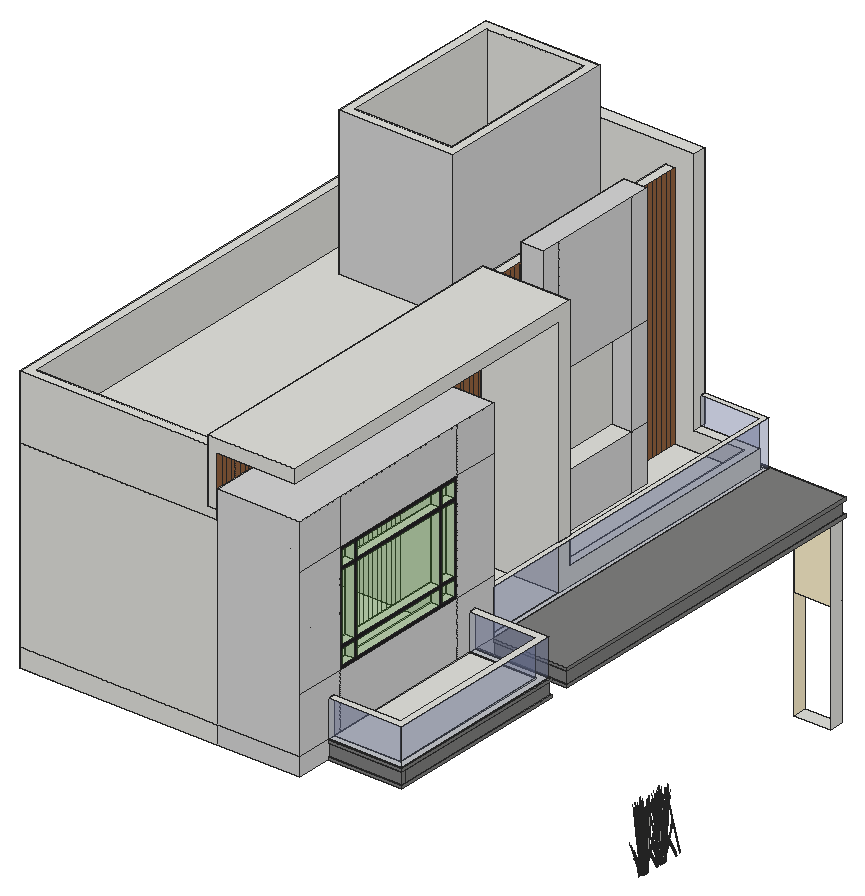
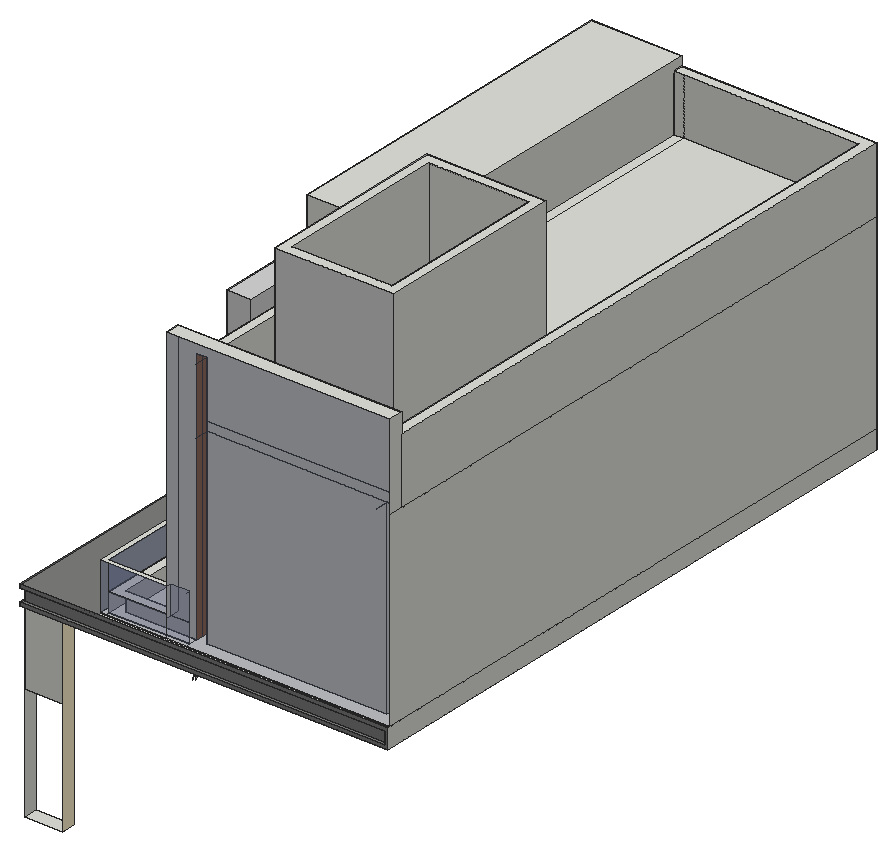
# SketchUp Ruby script. Lengths in inches.
U = 1.inch
M = Sketchup.active_model
def pt(a) = Geom::Point3d.new(a.map { |v| v * U })
def face(e, loops, mat)
  f = e.add_face(loops[0].map { |a| pt(a) })
  loops[1..].each { |l| e.add_face(l.map { |a| pt(a) }).erase! }
  f.material = f.back_material = mat if mat
  f
end
# faces: each face lists its corners as indices into pts; further lists are holes
def faces(e, pts, list, mat = nil) = list.each { |f| face(e, (f[0].is_a?(Array) ? f : [f]).map { |l| l.map { |i| pts[i] } }, mat) }
# xy, xz, yz: faces in a plane at the given z, y or x. An outline is a flat list of corners, or four numbers for a rectangle; further outlines are holes
def ring(l) = l.size == 4 ? [[l[0], l[1]], [l[2], l[1]], [l[2], l[3]], [l[0], l[3]]] : l.each_slice(2).to_a
def flat(e, list, mat, &to3) = list.each { |f| face(e, (f[0].is_a?(Array) ? f : [f]).map { |l| ring(l).map { |u, v| to3.(u, v) } }, mat) }
def xy(e, z, list, mat = nil) = flat(e, list, mat) { |x, y| [x, y, z] }
def xz(e, y, list, mat = nil) = flat(e, list, mat) { |x, z| [x, y, z] }
def yz(e, x, list, mat = nil) = flat(e, list, mat) { |y, z| [x, y, z] }
def lines(e, pts, list) = list.each { |a, b| e.add_line(pt(pts[a]), pt(pts[b])) }
# prism: a flat outline (further loops are holes) pulled along v
def prism(e, loops, v, mat = nil)
  f = face(e, loops, mat); d = Geom::Vector3d.new(v.map { |x| x * U })
  f.pushpull(f.normal.samedirection?(d) ? d.length : -d.length)
end
def box(e, o, s, mat = nil) = prism(e, [[o, [o[0] + s[0], o[1], o[2]], [o[0] + s[0], o[1] + s[1], o[2]], [o[0], o[1] + s[1], o[2]]]], [0, 0, s[2]], mat)
def at(x, y, z, deg = 0) = Geom::Transformation.translation(pt([x, y, z])) * Geom::Transformation.rotation(ORIGIN, Z_AXIS, deg.degrees)
def axes(o, x, y, z) = Geom::Transformation.new([*x, 0, *y, 0, *z, 0, *pt(o).to_a, 1])
def part(name) = M.definitions.add(name)
# library, detail: a bought-in or finely detailed component or shape, given as its bounding box
def library(name, o, s) = part(name).tap { |d| box(d.entities, o, s) }
def detail(e, o, s) = box(e.add_group.entities, o, s)
def put(e, d, t, mat = nil) = e.add_instance(d, t).tap { |i| i.material = mat if mat }
def group(e, t, mat = nil) = e.add_group.tap { |g| g.transformation = t; g.material = mat if mat }.entities
root = M.entities
M.materials.add("D01_Frost_White").color = [255, 242, 206]
M.materials.add("Glass_Basic_01").color = [81, 188, 38]
M.materials["Glass_Basic_01"].alpha = 0.25
M.materials.add("Glass_Sky Reflection_01").color = [126, 138, 183]
M.materials["Glass_Sky Reflection_01"].alpha = 0.25
M.materials.add("LightPink_Translucent").color = [144, 107, 117]
M.materials["LightPink_Translucent"].alpha = 0.75
M.materials.add("Marble_07_1K").color = [36, 34, 36]
M.materials.add("ThomThom - Waistcoat1").color = [214, 214, 214]
M.materials.add("ThomThom - Waistcoat2").color = [127, 127, 126]
M.materials.add("Wood_Veneer_15_1K").color = [150, 100, 65]
M.materials.add("wheel_emblem1").color = [204, 204, 204]
c1 = part("blade")
p = [[2.15,0.21,22],[0,0.17,0],[0.09,0.45,0],[2.18,0.31,22],[2.29,0.31,22],[0.38,0.45,0],
  [2.48,0.24,33],[2.49,0.24,33],[2.48,0.22,33]]
faces(c1.entities,p,[[0,1,2,3],[4,5,2,3],[6,3,4,7],[8,0,3,6]])
c2 = part("seeds")
p = [[0.3,-0.1,1.38],[-0.01,-0.03,1.59],[-0.01,-0.03,0.03],[0.14,-0.07,-0.07],[0.29,-0.03,3],[0.15,0.01,3.11]]
faces(c2.entities,p,[[0,1,2,3],[1,0,4,5]],"LightPink_Translucent")
c3 = part("blade with seeds")
put(c3.entities,c1,at(0,0,0))
put(c3.entities,c2,axes([2.4,0.25,30.99],[1.5799,-0.05474,1.17369],[-0.12525,1.92788,0.29478],[-0.07173,-0.02425,1.56792]))
g1 = group(root,at(0,1.43,120))
xy(g1,-120,[[207,375,231,384]])
xy(g1,0,[[207,375,231,384],[231,375,232,386],[207,384,231,386]])
xy(g1,0,[[0,0,183,24],[183,23,183,24,0,24,0,146.4,183,146.4,183,145,232,145,232,23],[0,146.4,183,150],[0,150,183,153.6],[0,153.6,183,157.2],
  [0,157.2,0,376.8,207,376.8,207,375,232,375,232,158,183,158,183,157.2],[0,376.8,207,380.4],[0,380.4,207,386]],"Wood_Veneer_15_1K")
xy(g1,2,[[183,23,231,24],[231,23,232,26],[231,26,232,145],[183,144,231,145],[231,158,232,158,232,386,2,386,2,384,231,384],
  [183,158,231,159]],"ThomThom - Waistcoat2")
xy(g1,6,[[183,28.5,226.5,139.5]])
xy(g1,10,[[183,23,231,24],[231,23,232,26]])
xy(g1,10,[[231,26,232,145],[183,144,231,145],[183,158,231,159],[231,158,232,386],[2,384,231,386]],"ThomThom - Waistcoat2")
xy(g1,12,[[[0,0,183,0,183,159,129,159,129,225,174,225,174,375,129,375,129,384,0,384],[129,249,144,333]],[183,24,231,24,231,144,183,144,183,139.5,226.5,139.5,226.5,28.5,183,28.5],[183,28.5,226.5,139.5],[129,159,180,216],[180,159,183,384],
  [129,216,180,216,180,249,174,249,174,225,129,225],[129,249,144,333],[174,249,180,333],[174,333,180,333,180,381,129,381,129,375,174,375],[129,381,180,384],
  [0,384,129,386],[129,384,141,386],[141,384,180,386],[180,384,183,386]])
xy(g1,12,[[183,23,231,24],[231,23,232,145],[183,144,231,145],[183,158,232,386]],"ThomThom - Waistcoat2")
xy(g1,24,[[174,225,180,225,180,381,141,381,141,375,174,375]])
xy(g1,36,[[183,24,231,24,231,144,183,144,183,139.5,226.5,139.5,226.5,28.5,183,28.5]])
xy(g1,42,[[180,159,183,159,183,384,141,384,141,381,180,381]])
xy(g1,48,[[129,261,130.78,321],[130.78,261,144,321]])
xy(g1,50,[[177,35,183,45],[177,47,183,115],[177,117,183,127]])
xy(g1,60,[[177,35,183,45],[177,47,183,115],[177,117,183,127]])
xy(g1,62,[[177,35,183,45],[177,47,183,115],[177,117,183,127]])
xy(g1,106,[[177,35,183,45],[177,47,183,115],[177,117,183,127]])
xy(g1,108,[[177,35,183,45],[177,47,183,115],[177,117,183,127],[129,261,130.78,321],[130.78,261,144,321]])
xy(g1,118,[[177,35,183,45],[177,47,183,115],[177,117,183,127]])
xy(g1,132,[[0,0,0,159,129,159,129,153,9,153,9,9,129,9,129,0],[9,9,129,153],[129,9,177,153],[0,159,9,375],[9,159,123,375]])
xy(g1,138,[[123,0,129,159],[117,6,123,6,123,375,6,375,6,369,117,369],[[6,6,117,369],[24,231,99,351]],[30,237,93,345]])
xy(g1,150,[[129,0,183,159]],"ThomThom - Waistcoat1")
xy(g1,171,[[129,0,180,216]],"Wood_Veneer_15_1K")
xy(g1,174,[[0,0,123,0,123,6,6,6,6,375,0,375],[123,225,129,375]])
xy(g1,180,[[123,0,180,225]])
xy(g1,186,[[0,375,141,384]])
xy(g1,186,[[129,249,144,333]],"ThomThom - Waistcoat1")
xy(g1,234,[[[24,231,99,351],[30,237,93,345]]])
xz(g1,0,[[0,0,129,12],[0,12,129,132],[0,132,129,132,129,138,123,138,123,174,0,174],[123,138,129,138,129,171,180,171,180,180,123,180]])
xz(g1,0,[[129,0,183,12],[129,12,183,150]],"ThomThom - Waistcoat1")
xz(g1,6,[[6,138,117,174],[117,138,123,174]])
xz(g1,9,[[9,12,177,132]])
xz(g1,23,[[183,0,232,2],[183,10,232,12]],"ThomThom - Waistcoat2")
xz(g1,24,[[183,12,231,36]],"Glass_Sky Reflection_01")
xz(g1,24,[[183,2,231,10]],"ThomThom - Waistcoat2")
xz(g1,28.5,[[183,6,226.5,12]])
xz(g1,28.5,[[183,12,226.5,36]],"Glass_Sky Reflection_01")
xz(g1,35,[[177,50,183,60],[177,62,183,106],[177,108,183,118]])
xz(g1,45,[[177,50,183,60],[177,62,183,106],[177,108,183,118]])
xz(g1,47,[[177,50,183,60],[177,62,183,106],[177,108,183,118]])
xz(g1,115,[[177,50,183,60],[177,62,183,106],[177,108,183,118]])
xz(g1,117,[[177,50,183,60],[177,62,183,106],[177,108,183,118]])
xz(g1,127,[[177,50,183,60],[177,62,183,106],[177,108,183,118]])
xz(g1,139.5,[[183,6,226.5,12]])
xz(g1,139.5,[[183,12,226.5,36]],"Glass_Sky Reflection_01")
xz(g1,144,[[183,12,231,36]],"Glass_Sky Reflection_01")
xz(g1,144,[[183,2,231,10]],"ThomThom - Waistcoat2")
xz(g1,145,[[183,0,232,2],[183,10,232,12]],"ThomThom - Waistcoat2")
xz(g1,153,[[9,12,177,132]])
xz(g1,158,[[183,0,232,2],[183,10,232,12]],"ThomThom - Waistcoat2")
xz(g1,159,[[9,12,123,132],[180,12,183,42],[123,132,129,138]])
xz(g1,159,[[129,12,129,150,183,150,183,42,180,42,180,12]],"ThomThom - Waistcoat1")
xz(g1,159,[[183,2,231,10]],"ThomThom - Waistcoat2")
xz(g1,216,[[129,12,180,171]])
xz(g1,225,[[129,12,129,174,123,174,123,180,180,180,180,24,174,24,174,12]])
xz(g1,231,[[24,138,99,234]],"ThomThom - Waistcoat1")
xz(g1,237,[[30,138,93,234]])
xz(g1,249,[[129,12,144,186]],"ThomThom - Waistcoat1")
xz(g1,261,[[129,48,130.78,108]])
xz(g1,261,[[130.78,48,144,108]],"ThomThom - Waistcoat1")
xz(g1,321,[[129,48,130.78,108]])
xz(g1,321,[[130.78,48,144,108]],"ThomThom - Waistcoat1")
xz(g1,333,[[129,12,144,186]],"ThomThom - Waistcoat1")
xz(g1,345,[[30,138,93,234]])
xz(g1,351,[[24,138,99,234]],"ThomThom - Waistcoat1")
xz(g1,375,[[129,12,174,12,174,24,141,24,141,186,0,186,0,174,6,174,6,138,123,138,123,174,129,174],[9,12,123,132],[0,132,123,132,123,138,6,138,6,174,0,174]])
xz(g1,375,[[207,-47.78,231,0]],"D01_Frost_White")
xz(g1,381,[[129,12,180,24],[129,24,141,42],[141,24,180,42]],"Glass_Sky Reflection_01")
xz(g1,384,[[207,-48,231,0]])
xz(g1,384,[[0,12,141,186],[141,12,183,42]],"Glass_Sky Reflection_01")
xz(g1,384,[[2,2,231,10]],"ThomThom - Waistcoat2")
xz(g1,386,[[0,0,0,12,232,12,232,10,2,10,2,2,232,2,232,0]],"ThomThom - Waistcoat2")
yz(g1,0,[[0,0,386,12],[0,12,384,132],[0,132,375,174],[375,132,384,186]])
yz(g1,2,[[384,2,386,10]],"ThomThom - Waistcoat2")
yz(g1,6,[[6,138,369,174],[369,138,375,174]])
yz(g1,9,[[9,12,153,132],[159,12,375,132]])
yz(g1,24,[[231,138,351,234]])
yz(g1,30,[[237,138,345,234]])
yz(g1,93,[[237,138,345,234]])
yz(g1,99,[[231,138,351,234]],"ThomThom - Waistcoat1")
yz(g1,123,[[159,12,375,132],[159,132,375,138],[0,138,6,174],[6,138,6,174,0,174,0,180,225,180,225,174,375,174,375,138]])
yz(g1,129,[[216,12,225,174],[249,12,262.5,12,262.5,48,261,48,261,108,321,108,321,48,318.75,48,318.75,12,333,12,333,174,249,174],[262.5,12,266.25,48],[266.25,12,270,48],[270,12,273.75,48],
  [273.75,12,277.5,48],[277.5,12,281.25,48],[281.25,12,285,48],[285,12,288.75,48],[288.75,12,292.5,48],
  [292.5,12,296.25,48],[296.25,12,300,48],[300,12,303.75,48],[303.75,12,307.5,48],[307.5,12,311.25,48],
  [311.25,12,315,48],[315,12,318.75,48],[0,132,3.75,138],[3.75,132,7.5,138],[7.5,132,11.25,138],
  [11.25,132,15,138],[15,132,18.75,138],[18.75,132,22.5,138],[22.5,132,26.25,138],[26.25,132,30,138],
  [30,132,33.75,138],[33.75,132,37.5,138],[37.5,132,41.25,138],[41.25,132,45,138],[45,132,48.75,138],
  [48.75,132,52.5,138],[52.5,132,56.25,138],[56.25,132,60,138],[60,132,63.75,138],[63.75,132,67.5,138],
  [67.5,132,71.25,138],[71.25,132,75,138],[75,132,78.75,138],[78.75,132,82.5,138],[82.5,132,86.25,138],
  [86.25,132,90,138],[90,132,93.75,138],[93.75,132,97.5,138],[97.5,132,101.25,138],[101.25,132,105,138],
  [105,132,108.75,138],[108.75,132,112.5,138],[112.5,132,116.25,138],[116.25,132,120,138],[120,132,123.75,138],
  [123.75,132,127.5,138],[127.5,132,131.25,138],[131.25,132,135,138],[135,132,138.75,138],[138.75,132,142.5,138],
  [142.5,132,146.25,138],[146.25,132,150,138],[150,132,153.75,138],[153.75,132,157.5,138],[157.5,132,159,138],
  [0,138,3.75,150],[3.75,138,7.5,150],[7.5,138,11.25,150],[11.25,138,15,150],[15,138,18.75,150],
  [18.75,138,22.5,150],[22.5,138,26.25,150],[26.25,138,30,150],[30,138,33.75,150],[33.75,138,37.5,150],
  [37.5,138,41.25,150],[41.25,138,45,150],[45,138,48.75,150],[48.75,138,52.5,150],[52.5,138,56.25,150],
  [56.25,138,60,150],[60,138,63.75,150],[63.75,138,67.5,150],[67.5,138,71.25,150],[71.25,138,75,150],
  [75,138,78.75,150],[78.75,138,82.5,150],[82.5,138,86.25,150],[86.25,138,90,150],[90,138,93.75,150],
  [93.75,138,97.5,150],[97.5,138,101.25,150],[101.25,138,105,150],[105,138,108.75,150],[108.75,138,112.5,150],
  [112.5,138,116.25,150],[116.25,138,120,150],[120,138,123.75,150],[123.75,138,127.5,150],[127.5,138,131.25,150],
  [131.25,138,135,150],[135,138,138.75,150],[138.75,138,142.5,150],[142.5,138,146.25,150],[146.25,138,150,150],
  [150,138,153.75,150],[153.75,138,157.5,150],[157.5,138,159,150]])
yz(g1,129,[[249,174,333,186]],"ThomThom - Waistcoat1")
yz(g1,129,[[159,12,161.25,12,161.25,171,157.5,171,157.5,150,159,150],[161.25,12,165,171],[165,12,168.75,171],[168.75,12,172.5,171],[172.5,12,176.25,171],
  [176.25,12,180,171],[180,12,183.75,171],[183.75,12,187.5,171],[187.5,12,191.25,171],[191.25,12,195,171],
  [195,12,198.75,171],[198.75,12,202.5,171],[202.5,12,206.25,171],[206.25,12,210,171],[210,12,213.75,171],
  [213.75,12,216,171],[225,12,249,174],[333,12,375,174],[0,150,3.75,171],[3.75,150,7.5,171],
  [7.5,150,11.25,171],[11.25,150,15,171],[15,150,18.75,171],[18.75,150,22.5,171],[22.5,150,26.25,171],
  [26.25,150,30,171],[30,150,33.75,171],[33.75,150,37.5,171],[37.5,150,41.25,171],[41.25,150,45,171],
  [45,150,48.75,171],[48.75,150,52.5,171],[52.5,150,56.25,171],[56.25,150,60,171],[60,150,63.75,171],
  [63.75,150,67.5,171],[67.5,150,71.25,171],[71.25,150,75,171],[75,150,78.75,171],[78.75,150,82.5,171],
  [82.5,150,86.25,171],[86.25,150,90,171],[90,150,93.75,171],[93.75,150,97.5,171],[97.5,150,101.25,171],
  [101.25,150,105,171],[105,150,108.75,171],[108.75,150,112.5,171],[112.5,150,116.25,171],[116.25,150,120,171],
  [120,150,123.75,171],[123.75,150,127.5,171],[127.5,150,131.25,171],[131.25,150,135,171],[135,150,138.75,171],
  [138.75,150,142.5,171],[142.5,150,146.25,171],[146.25,150,150,171],[150,150,153.75,171],[153.75,150,157.5,171]],"Wood_Veneer_15_1K")
yz(g1,130.78,[[261,48,321,108]])
yz(g1,141,[[375,24,381,24,381,42,384,42,384,186,375,186],[381,24,384,42]])
yz(g1,144,[[249,12,261,48],[261,12,321,48],[321,12,333,48],[249,48,261,108],[321,48,333,108],
  [249,108,261,186],[261,108,321,186],[321,108,333,186]],"ThomThom - Waistcoat1")
yz(g1,174,[[225,12,375,24]])
yz(g1,177,[[[9,12,153,132],[47,62,115,62,115,106,47,106,47,108,115,108,115,118,47,118],[47,50,115,60],[35,62,45,106],[117,62,127,106],[35,108,45,118],[117,108,127,118],[117,50,127,60],[35,50,45,60]]])
yz(g1,180,[[216,12,381,12,381,24,225,24,225,42,216,42],[216,42,225,42,225,180,0,180,0,171,216,171]])
yz(g1,180,[[159,12,216,42],[225,24,381,42]],"Glass_Sky Reflection_01")
yz(g1,183,[[28.5,6,139.5,12],[24,12,28.5,36],[139.5,12,144,36]])
yz(g1,183,[[35,50,45,60],[47,50,115,60],[117,50,127,60],[35,62,45,106],[47,62,115,106],
  [117,62,127,106],[35,108,45,118],[47,108,115,118],[117,108,127,118]],"Glass_Basic_01")
yz(g1,183,[[159,12,384,42]],"Glass_Sky Reflection_01")
yz(g1,183,[[[33,48,129,120],[47,62,115,106],[35,50,35,118,127,118,127,50,47,50,47,60,115,60,115,50,117,50,117,60,127,60,127,62,117,62,117,106,127,106,127,108,117,108,117,118,115,118,115,108,47,108,47,118,45,118,45,108,35,108,35,106,45,106,45,62,35,62,35,60,45,60,45,50]]],"Marble_07_1K")
yz(g1,183,[[0,0,23,0,23,2,24,2,24,10,23,10,23,12,0,12],[0,12,24,12,24,36,28.5,36,28.5,12,33,12,33,48,0,48],[33,12,129,48],[129,12,139.5,12,139.5,36,144,36,144,12,159,12,159,48,129,48],[0,48,33,120],
  [129,48,159,120],[0,120,33,150],[33,120,129,150],[129,120,159,150]],"ThomThom - Waistcoat1")
yz(g1,183,[[145,0,158,0,158,2,159,2,159,10,158,10,158,12,145,12,145,10,144,10,144,2,145,2]],"wheel_emblem1")
yz(g1,207,[[375,-120,384,0]],"D01_Frost_White")
yz(g1,226.5,[[28.5,6,139.5,12]])
yz(g1,226.5,[[28.5,12,139.5,36]],"Glass_Sky Reflection_01")
yz(g1,231,[[375,-120,384,0]])
yz(g1,231,[[24,12,144,36]],"Glass_Sky Reflection_01")
yz(g1,231,[[24,2,26,10],[26,2,144,10],[159,2,384,10]],"ThomThom - Waistcoat2")
yz(g1,232,[[23,0,145,2],[158,0,386,2],[23,10,145,12],[158,10,386,12]],"ThomThom - Waistcoat2")
p = [[177,9,12],[183,9,12],[129,159,138],[129.2,159,138],[129,381,42],[129,384,42],
  [122.18,159,138],[123,159,138],[123,375,174],[123,384,174],[123,375,132],[123,384,132],
  [9,384,132],[9,375,132],[177,9,84],[183,9,84],[180,219,12],[180.01,219,12],
  [177,9,132],[177,0,132],[177,47,108],[177,45,108],[177,47,106],[177,45,106],
  [231,384,-48],[207,375,-47.78],[129,371.25,11.97],[129,371.25,12],[129,371.25,173.97],[129,367.5,11.94],
  [129,367.5,12],[129,367.5,173.94],[129,363.75,11.91],[129,363.75,12],[129,363.75,173.91],[129,360,11.88],
  [129,360,12],[129,360,173.88],[129,356.25,11.85],[129,356.25,12],[129,356.25,173.85],[129,352.5,11.82],
  [129,352.5,12],[129,352.5,173.82],[129,348.75,11.79],[129,348.75,12],[129,348.75,173.79],[129,345,11.76],
  [129,345,12],[129,345,173.76],[129,341.25,11.73],[129,341.25,12],[129,341.25,173.73],[129,337.5,11.7],
  [129,337.5,12],[129,337.5,173.7],[129,333.75,11.67],[129,333.75,12],[129,333.75,173.67],[129,330,11.64],
  [129,330,12],[129,330,173.64],[129,326.25,11.61],[129,326.25,12],[129,326.25,173.61],[129,322.5,11.58],
  [129,322.5,12],[129,322.5,173.58],[129,318.75,11.55],[129,318.75,12],[129,318.75,48],[129,318.75,108],
  [129,318.75,173.55],[129,315,11.52],[129,315,12],[129,315,48],[129,315,108],[129,315,173.52],
  [129,311.25,11.49],[129,311.25,12],[129,311.25,108],[129,311.25,173.49],[129,311.25,48],[129,307.5,11.46],
  [129,307.5,12],[129,307.5,108],[129,307.5,173.46],[129,307.5,48],[129,303.75,11.43],[129,303.75,12],
  [129,303.75,48],[129,303.75,108],[129,303.75,173.43],[129,300,11.4],[129,300,12],[129,300,48],
  [129,300,108],[129,300,173.4],[129,296.25,11.37],[129,296.25,12],[129,296.25,48],[129,296.25,108],
  [129,296.25,173.37],[129,292.5,11.34],[129,292.5,12],[129,292.5,48],[129,292.5,108],[129,292.5,173.34],
  [129,288.75,11.31],[129,288.75,12],[129,288.75,48],[129,288.75,108],[129,288.75,173.31],[129,285,11.28],
  [129,285,12],[129,285,48],[129,285,108],[129,285,173.28],[129,281.25,11.25],[129,281.25,12],
  [129,281.25,48],[129,281.25,108],[129,281.25,173.25],[129,277.5,11.22],[129,277.5,12],[129,277.5,48],
  [129,277.5,108],[129,277.5,173.22],[129,273.75,11.19],[129,273.75,12],[129,273.75,48],[129,273.75,108],
  [129,273.75,173.19],[129,270,11.16],[129,270,12],[129,270,108],[129,270,173.16],[129,270,48],
  [129,266.25,11.13],[129,266.25,12],[129,266.25,108],[129,266.25,173.13],[129,266.25,48],[129,262.5,11.1],
  [129,262.5,12],[129,262.5,48],[129,262.5,108],[129,262.5,173.1],[129,258.75,11.07],[129,258.75,12],
  [129,258.75,173.07],[129,255,11.04],[129,255,12],[129,255,173.04],[129,251.25,11.01],[129,251.25,12],
  [129,251.25,173.01],[129,247.5,10.98],[129,247.5,12],[129,247.5,172.98],[129,243.75,10.95],[129,243.75,12],
  [129,243.75,172.95],[129,240,10.92],[129,240,12],[129,240,172.92],[129,236.25,10.89],[129,236.25,12],
  [129,236.25,172.89],[129,232.5,10.86],[129,232.5,12],[129,232.5,172.86],[129,228.75,10.83],[129,228.75,12],
  [129,228.75,172.83],[129,225,10.8],[129,225,12],[129,221.25,10.77],[129,221.25,12],[129,221.25,172.77],
  [129,217.5,10.74],[129,217.5,12],[129,217.5,172.74],[129,213.75,10.71],[129,213.75,12],[129,213.75,171],
  [129,213.75,172.71],[129,210,10.68],[129,210,12],[129,210,171],[129,210,172.68],[129,206.25,10.65],
  [129,206.25,12],[129,206.25,171],[129,206.25,172.65],[129,202.5,10.62],[129,202.5,12],[129,202.5,171],
  [129,202.5,172.62],[129,198.75,10.59],[129,198.75,12],[129,198.75,171],[129,198.75,172.59],[129,195,10.56],
  [129,195,12],[129,195,171],[129,195,172.56],[129,191.25,10.53],[129,191.25,12],[129,191.25,171],
  [129,191.25,172.53],[129,187.5,10.5],[129,187.5,12],[129,187.5,171],[129,187.5,172.5],[129,183.75,10.47],
  [129,183.75,12],[129,183.75,171],[129,183.75,172.47],[129,180,10.44],[129,180,12],[129,180,171],
  [129,180,172.44],[129,176.25,10.41],[129,176.25,12],[129,176.25,171],[129,176.25,172.41],[129,172.5,10.38],
  [129,172.5,12],[129,172.5,171],[129,172.5,172.38],[129,168.75,10.35],[129,168.75,12],[129,168.75,171],
  [129,168.75,172.35],[129,165,10.32],[129,165,12],[129,165,171],[129,165,172.32],[129,161.25,10.29],
  [129,161.25,12],[129,161.25,171],[129,161.25,172.29],[129,157.5,10.26],[129,157.5,132],[129,157.5,171],
  [129,157.5,172.26],[129,153.75,10.23],[129,153.75,132],[129,153.75,171],[129,153.75,172.23],[129,150,10.2],
  [129,150,132],[129,150,171],[129,150,172.2],[129,146.25,10.17],[129,146.25,132],[129,146.25,171],
  [129,146.25,172.17],[129,142.5,10.14],[129,142.5,132],[129,142.5,171],[129,142.5,172.14],[129,138.75,10.11],
  [129,138.75,132],[129,138.75,171],[129,138.75,172.11],[129,135,10.08],[129,135,132],[129,135,171],
  [129,135,172.08],[129,131.25,10.05],[129,131.25,132],[129,131.25,171],[129,131.25,172.05],[129,127.5,10.02],
  [129,127.5,132],[129,127.5,171],[129,127.5,172.02],[129,123.75,9.99],[129,123.75,132],[129,123.75,171],
  [129,123.75,171.99],[129,120,9.96],[129,120,132],[129,120,171],[129,120,171.96],[129,116.25,9.93],
  [129,116.25,132],[129,116.25,171],[129,116.25,171.93],[129,112.5,9.9],[129,112.5,132],[129,112.5,171],
  [129,112.5,171.9],[129,108.75,9.87],[129,108.75,132],[129,108.75,171],[129,108.75,171.87],[129,105,9.84],
  [129,105,132],[129,105,171],[129,105,171.84],[129,101.25,9.81],[129,101.25,132],[129,101.25,171],
  [129,101.25,171.81],[129,97.5,9.78],[129,97.5,132],[129,97.5,171],[129,97.5,171.78],[129,93.75,9.75],
  [129,93.75,132],[129,93.75,171],[129,93.75,171.75],[129,90,9.72],[129,90,132],[129,90,171],
  [129,90,171.72],[129,86.25,9.69],[129,86.25,132],[129,86.25,171],[129,86.25,171.69],[129,82.5,9.66],
  [129,82.5,132],[129,82.5,171],[129,82.5,171.66],[129,78.75,9.63],[129,78.75,132],[129,78.75,171],
  [129,78.75,171.63],[129,75,9.6],[129,75,132],[129,75,171],[129,75,171.6],[129,71.25,9.57],
  [129,71.25,132],[129,71.25,171],[129,71.25,171.57],[129,67.5,9.54],[129,67.5,132],[129,67.5,171],
  [129,67.5,171.54],[129,63.75,9.51],[129,63.75,132],[129,63.75,171],[129,63.75,171.51],[129,60,9.48],
  [129,60,132],[129,60,171],[129,60,171.48],[129,56.25,9.45],[129,56.25,132],[129,56.25,171],
  [129,56.25,171.45],[129,52.5,9.42],[129,52.5,132],[129,52.5,171],[129,52.5,171.42],[129,48.75,9.39],
  [129,48.75,132],[129,48.75,171],[129,48.75,171.39],[129,45,9.36],[129,45,132],[129,45,171],
  [129,45,171.36],[129,41.25,9.33],[129,41.25,132],[129,41.25,171],[129,41.25,171.33],[129,37.5,9.3],
  [129,37.5,132],[129,37.5,171],[129,37.5,171.3],[129,33.75,9.27],[129,33.75,132],[129,33.75,171],
  [129,33.75,171.27],[129,30,9.24],[129,30,132],[129,30,171],[129,30,171.24],[129,26.25,9.21],
  [129,26.25,132],[129,26.25,171],[129,26.25,171.21],[129,22.5,9.18],[129,22.5,132],[129,22.5,171],
  [129,22.5,171.18],[129,18.75,9.15],[129,18.75,132],[129,18.75,171],[129,18.75,171.15],[129,15,9.12],
  [129,15,132],[129,15,171],[129,15,171.12],[129,11.25,9.09],[129,11.25,132],[129,11.25,171],
  [129,11.25,171.09],[129,7.5,9.06],[129,7.5,132],[129,7.5,171],[129,7.5,171.06],[129,3.75,9.03],
  [129,3.75,132],[129,3.75,171],[129,3.75,171.03],[207,373.2,0],[0,373.2,0],[207,369.6,0],
  [0,369.6,0],[207,366,0],[0,366,0],[207,362.4,0],[0,362.4,0],[207,358.8,0],
  [0,358.8,0],[207,355.2,0],[0,355.2,0],[207,351.6,0],[0,351.6,0],[207,348,0],
  [0,348,0],[207,344.4,0],[0,344.4,0],[207,340.8,0],[0,340.8,0],[207,337.2,0],
  [0,337.2,0],[207,333.6,0],[0,333.6,0],[207,330,0],[0,330,0],[207,326.4,0],
  [0,326.4,0],[207,322.8,0],[0,322.8,0],[207,319.2,0],[0,319.2,0],[207,315.6,0],
  [0,315.6,0],[207,312,0],[0,312,0],[207,308.4,0],[0,308.4,0],[207,304.8,0],
  [0,304.8,0],[207,301.2,0],[0,301.2,0],[207,297.6,0],[0,297.6,0],[207,294,0],
  [0,294,0],[207,290.4,0],[0,290.4,0],[207,286.8,0],[0,286.8,0],[207,283.2,0],
  [0,283.2,0],[207,279.6,0],[0,279.6,0],[207,276,0],[0,276,0],[207,272.4,0],
  [0,272.4,0],[207,268.8,0],[0,268.8,0],[207,265.2,0],[0,265.2,0],[207,261.6,0],
  [0,261.6,0],[207,258,0],[0,258,0],[207,254.4,0],[0,254.4,0],[207,250.8,0],
  [0,250.8,0],[207,247.2,0],[0,247.2,0],[207,243.6,0],[0,243.6,0],[207,240,0],
  [0,240,0],[207,236.4,0],[0,236.4,0],[207,232.8,0],[0,232.8,0],[207,229.2,0],
  [0,229.2,0],[207,225.6,0],[0,225.6,0],[207,222,0],[0,222,0],[207,218.4,0],
  [0,218.4,0],[207,214.8,0],[0,214.8,0],[207,211.2,0],[0,211.2,0],[207,207.6,0],
  [0,207.6,0],[207,204,0],[0,204,0],[207,200.4,0],[0,200.4,0],[207,196.8,0],
  [0,196.8,0],[207,193.2,0],[0,193.2,0],[207,189.6,0],[0,189.6,0],[207,186,0],
  [0,186,0],[207,182.4,0],[0,182.4,0],[207,178.8,0],[0,178.8,0],[207,175.2,0],
  [0,175.2,0],[207,171.6,0],[0,171.6,0],[207,168,0],[0,168,0],[207,164.4,0],
  [0,164.4,0],[207,160.8,0],[0,160.8,0],[207,142.8,0],[0,142.8,0],[207,139.2,0],
  [0,139.2,0],[207,135.6,0],[0,135.6,0],[207,132,0],[0,132,0],[207,128.4,0],
  [0,128.4,0],[207,124.8,0],[0,124.8,0],[207,121.2,0],[0,121.2,0],[207,117.6,0],
  [0,117.6,0],[207,114,0],[0,114,0],[207,110.4,0],[0,110.4,0],[207,106.8,0],
  [0,106.8,0],[207,103.2,0],[0,103.2,0],[207,99.6,0],[0,99.6,0],[207,96,0],
  [0,96,0],[207,92.4,0],[0,92.4,0],[207,88.8,0],[0,88.8,0],[207,85.2,0],
  [0,85.2,0],[207,81.6,0],[0,81.6,0],[207,78,0],[0,78,0],[207,74.4,0],
  [0,74.4,0],[207,70.8,0],[0,70.8,0],[207,67.2,0],[0,67.2,0],[207,63.6,0],
  [0,63.6,0],[207,60,0],[0,60,0],[207,56.4,0],[0,56.4,0],[207,52.8,0],
  [0,52.8,0],[207,49.2,0],[0,49.2,0],[207,45.6,0],[0,45.6,0],[207,42,0],
  [0,42,0],[207,38.4,0],[0,38.4,0],[207,34.8,0],[0,34.8,0],[207,31.2,0],
  [0,31.2,0],[207,27.6,0],[0,27.6,0]]
lines(g1,p,[[0,1],[2,3],[4,5],[6,7],[8,9],[10,11],[12,13],[14,15],[16,17],[18,19],[20,21],[22,23],
  [21,23],[24,25],[26,27],[27,28],[29,30],[30,31],[32,33],[33,34],[35,36],[36,37],[38,39],[39,40],
  [41,42],[42,43],[44,45],[45,46],[47,48],[48,49],[50,51],[51,52],[53,54],[54,55],[56,57],[57,58],
  [59,60],[60,61],[62,63],[63,64],[65,66],[66,67],[68,69],[70,71],[71,72],[73,74],[75,76],[76,77],
  [78,79],[80,81],[82,80],[83,84],[85,86],[87,85],[88,89],[90,91],[91,92],[93,94],[95,96],[96,97],
  [98,99],[100,101],[101,102],[103,104],[105,106],[106,107],[108,109],[110,111],[111,112],[113,114],[115,116],[116,117],
  [118,119],[120,121],[121,122],[123,124],[125,126],[126,127],[128,129],[130,131],[131,132],[133,134],[135,136],[137,135],
  [138,139],[140,141],[142,140],[143,144],[145,146],[146,147],[148,149],[149,150],[151,152],[152,153],[154,155],[155,156],
  [157,158],[158,159],[160,161],[161,162],[163,164],[164,165],[166,167],[167,168],[169,170],[170,171],[172,173],[173,174],
  [175,176],[177,178],[178,179],[180,181],[181,182],[183,184],[185,186],[187,188],[189,190],[191,192],[193,194],[195,196],
  [197,198],[199,200],[201,202],[203,204],[205,206],[207,208],[209,210],[211,212],[213,214],[215,216],[217,218],[219,220],
  [221,222],[223,224],[225,226],[227,228],[229,230],[231,232],[233,234],[235,236],[237,238],[239,240],[241,242],[243,244],
  [245,246],[247,248],[249,250],[251,252],[253,254],[255,256],[257,258],[259,260],[261,262],[263,264],[265,266],[267,268],
  [269,270],[271,272],[273,274],[275,276],[277,278],[279,280],[281,282],[283,284],[285,286],[287,288],[289,290],[291,292],
  [293,294],[295,296],[297,298],[299,300],[301,302],[303,304],[305,306],[307,308],[309,310],[311,312],[313,314],[315,316],
  [317,318],[319,320],[321,322],[323,324],[325,326],[327,328],[329,330],[331,332],[333,334],[335,336],[337,338],[339,340],
  [341,342],[343,344],[345,346],[347,348],[349,350],[351,352],[353,354],[355,356],[357,358],[359,360],[361,362],[363,364],
  [365,366],[367,368],[369,370],[371,372],[373,374],[375,376],[377,378],[379,380],[381,382],[383,384],[385,386],[387,388],
  [389,390],[391,392],[393,394],[395,396],[397,398],[399,400],[401,402],[403,404],[405,406],[407,408],[409,410],[411,412],
  [413,414],[415,416],[417,418],[419,420],[421,422],[423,424],[425,426],[427,428],[429,430],[431,432],[433,434],[435,436],
  [437,438],[439,440],[441,442],[443,444],[445,446],[447,448],[449,450],[451,452],[453,454],[455,456],[457,458],[459,460],
  [461,462],[463,464],[465,466],[467,468],[469,470],[471,472],[473,474],[475,476],[477,478],[479,480],[481,482],[483,484],
  [485,486],[487,488],[489,490],[491,492],[493,494],[495,496],[497,498],[499,500],[501,502],[503,504],[505,506],[507,508],
  [509,510],[511,512],[513,514],[515,516],[517,518],[519,520],[521,522],[523,524],[525,526],[527,528],[529,530],[531,532],
  [533,534],[535,536],[537,538],[539,540],[541,542],[543,544],[545,546],[547,548],[549,550],[551,552],[553,554],[555,556],
  [557,558],[559,560],[561,562],[563,564],[565,566],[567,568],[569,570],[571,572],[573,574],[575,576],[577,578],[579,580],
  [581,582],[583,584],[585,586],[587,588],[589,590],[591,592],[593,594],[595,596]])
put(root,c3,axes([250.27,198.28,1.07],[0.08895,0.05019,1.03788],[0.05733,0.5127,-0.22321],[-0.12083,0.09597,0.44375]))
put(root,c3,axes([250.27,213.53,1.07],[0.08895,0.05019,1.03788],[0.05733,0.5127,-0.22321],[-0.12083,0.09597,0.44375]))
put(root,c3,axes([250.62,195.8,1.07],[0.04997,0.17024,1.03788],[-0.11515,0.46273,-0.22321],[-0.11824,-0.1106,0.44375]))
put(root,c3,axes([250.62,211.05,1.07],[0.04997,0.17024,1.03788],[-0.11515,0.46273,-0.22321],[-0.11824,-0.1106,0.44375]))
put(root,c3,axes([250.44,196.9375,0.28],[0.00649,0.09636,1.27986],[-0.13086,0.50324,-0.19552],[-0.09295,-0.02537,0.218]))
put(root,c3,axes([250.44,212.19,0.28],[0.00649,0.09636,1.27986],[-0.13086,0.50324,-0.19552],[-0.09295,-0.02537,0.218]))
put(root,c3,axes([250.09,199.35,1.2],[0.10667,-0.27712,0.83364],[0.04209,0.43871,0.6125],[-0.07709,0.07855,0.18362]))
put(root,c3,axes([250.09,214.6,1.2],[0.10667,-0.27712,0.83364],[0.04209,0.43871,0.6125],[-0.07709,0.07855,0.18362]))
put(root,c3,axes([250.37,199.64,0.28],[0.03433,0.06109,1.27986],[0.05822,0.56601,-0.19552],[-0.07609,0.1207,0.218]))
put(root,c3,axes([250.37,214.89,0.28],[0.03433,0.06109,1.27986],[0.05822,0.56601,-0.19552],[-0.07609,0.1207,0.218]))
put(root,c3,axes([250.32,196.31,1.2],[0.16341,-0.04375,0.83364],[-0.10366,0.38551,0.6125],[-0.08075,-0.05783,0.18362]))
put(root,c3,axes([250.32,211.56,1.2],[0.16341,-0.04375,0.83364],[-0.10366,0.38551,0.6125],[-0.08075,-0.05783,0.18362]))
put(root,c3,axes([251.3,197.8125,0.6875],[-0.26625,-0.10025,-0.45255],[0.05619,-0.61836,-0.11877],[-0.07946,-0.07493,0.99892]))
put(root,c3,axes([251.3,213.0625,0.6875],[-0.26625,-0.10025,-0.45255],[0.05619,-0.61836,-0.11877],[-0.07946,-0.07493,0.99892]))
put(root,c3,axes([250.95,198.98,0.66],[-0.23955,-0.30573,-0.36036],[0.14318,-0.54821,0],[-0.05456,-0.06963,1.14313]))
put(root,c3,axes([250.95,214.23,0.66],[-0.23955,-0.30573,-0.36036],[0.14318,-0.54821,0],[-0.05456,-0.06963,1.14313]))
put(root,c3,axes([250.84,209.68,0.28],[-0.02479,0.08055,1.27986],[-0.25056,0.17367,-0.19552],[-0.06053,-0.15798,0.218]))
put(root,c3,axes([250.84,225.19,0.28],[-0.02479,0.08055,1.27986],[-0.25056,0.17367,-0.19552],[-0.06053,-0.15798,0.218]))
put(root,c3,axes([251.09,199.35,0.91],[-0.16003,0.61271,0],[-0.26773,-0.34169,-0.37456],[-0.06098,-0.07782,1.18819]))
put(root,c3,axes([251.09,214.6,0.91],[-0.16003,0.61271,0],[-0.26773,-0.34169,-0.37456],[-0.06098,-0.07782,1.18819]))
put(root,c3,axes([250.8,200.24,1.07],[0.08077,-0.09646,1.03788],[0.19942,0.29084,-0.22321],[-0.05936,0.25166,0.44375]))
put(root,c3,axes([250.8,215.49,1.07],[0.08077,-0.09646,1.03788],[0.19942,0.29084,-0.22321],[-0.05936,0.25166,0.44375]))
put(root,c3,axes([250.6875,194.74,0.74],[-0.07384,0.49928,-0.02825],[-0.22725,-0.15358,-0.1281],[-0.0345,-0.08166,0.42251]))
put(root,c3,axes([250.6875,209.99,0.74],[-0.07384,0.49928,-0.02825],[-0.22725,-0.15358,-0.1281],[-0.0345,-0.08166,0.42251]))
put(root,c3,axes([251.03,209.36,1.07],[-0.0155,0.20002,1.03788],[-0.22659,0.16744,-0.22321],[-0.05297,-0.25854,0.44375]))
put(root,c3,axes([251.03,224.87,1.07],[-0.0155,0.20002,1.03788],[-0.22659,0.16744,-0.22321],[-0.05297,-0.25854,0.44375]))
put(root,c3,axes([251.6,197.9,1.13],[-0.25843,0.40595,-0.21117],[-0.17185,-0.5736,-0.36291],[-0.06376,-0.05825,1.15913]))
put(root,c3,axes([251.6,213.16,1.13],[-0.25843,0.40595,-0.21117],[-0.17185,-0.5736,-0.36291],[-0.06376,-0.05825,1.15913]))
put(root,c3,axes([250.5625,197.02,0.91],[-0.32006,0,0],[0,-0.68339,-0.37456],[0,-0.15565,1.18819]))
put(root,c3,axes([250.5625,212.27,0.91],[-0.32006,0,0],[0,-0.68339,-0.37456],[0,-0.15565,1.18819]))
put(root,c3,axes([251.01,198.75,0.66],[-0.06012,-0.53279,-0.22483],[0.23879,-0.15129,0.22483],[-0.04814,-0.06144,1.00865]))
put(root,c3,axes([251.01,214.01,0.66],[-0.06012,-0.53279,-0.22483],[0.23879,-0.15129,0.22483],[-0.04814,-0.06144,1.00865]))
put(root,c3,axes([251.77,198.35,0.6875],[-0.1724,0.45959,-0.45255],[-0.21416,-0.41674,-0.11877],[-0.06908,0.11465,0.99892]))
put(root,c3,axes([251.77,213.6,0.6875],[-0.1724,0.45959,-0.45255],[-0.21416,-0.41674,-0.11877],[-0.06908,0.11465,0.99892]))
put(root,c3,axes([250.8125,196.84,0.88],[-0.23808,0.51407,0.22322],[-0.23822,-0.50866,-0.26485],[-0.00831,-0.14599,1.19671]))
put(root,c3,axes([250.8125,212.09,0.88],[-0.23808,0.51407,0.22322],[-0.23822,-0.50866,-0.26485],[-0.00831,-0.14599,1.19671]))
put(root,c3,axes([250.95,209.04,1.2],[0.13352,0.21281,0.83364],[-0.19445,0.12793,0.6125],[-0.0416,-0.16355,0.18362]))
put(root,c3,axes([250.95,224.55,1.2],[0.13352,0.21281,0.83364],[-0.19445,0.12793,0.6125],[-0.0416,-0.16355,0.18362]))
put(root,c3,axes([251.89,198.09,0.98],[-0.24993,-0.49214,-0.18284],[0.21031,-0.55263,0.40012],[-0.0673,0.05757,1.22088]))
put(root,c3,axes([251.89,213.34,0.98],[-0.24993,-0.49214,-0.18284],[0.21031,-0.55263,0.40012],[-0.0673,0.05757,1.22088]))
put(root,c3,axes([251.43,197.61,0.8],[-0.15376,-0.51322,-0.32471],[0.2329,-0.3614,0.15627],[-0.04976,-0.0635,1.04254]))
put(root,c3,axes([251.43,212.87,0.8],[-0.15376,-0.51322,-0.32471],[0.2329,-0.3614,0.15627],[-0.04976,-0.0635,1.04254]))
put(root,c3,axes([250.99,200.5625,1.2],[-0.00662,-0.36357,0.83364],[0.16552,0.25931,0.6125],[-0.03255,0.17329,0.18362]))
put(root,c3,axes([250.99,215.8125,1.2],[-0.00662,-0.36357,0.83364],[0.16552,0.25931,0.6125],[-0.03255,0.17329,0.18362]))
put(root,c3,axes([251.76,197.98,0.8],[-0.27795,0.03775,-0.32471],[-0.02514,-0.62656,0.15627],[-0.04976,0.0635,1.04254]))
put(root,c3,axes([251.76,213.24,0.8],[-0.27795,0.03775,-0.32471],[-0.02514,-0.62656,0.15627],[-0.04976,0.0635,1.04254]))
put(root,c3,axes([251.23,199.03,0.99],[0.23955,0.30573,0.36036],[-0.14318,0.54821,0],[-0.05456,-0.06963,1.14313]))
put(root,c3,axes([251.23,214.28,0.99],[0.23955,0.30573,0.36036],[-0.14318,0.54821,0],[-0.05456,-0.06963,1.14313]))
put(root,c3,axes([251.46,197.91,0.96],[0.06784,-0.72454,-0.17004],[0.32166,0.1263,0.37211],[-0.05621,-0.10006,1.13542]))
put(root,c3,axes([251.46,213.16,0.96],[0.06784,-0.72454,-0.17004],[0.32166,0.1263,0.37211],[-0.05621,-0.10006,1.13542]))
put(root,c3,axes([251.57,198.08,1.09],[-0.04938,0.54569,0.10509],[-0.24125,-0.09472,-0.30009],[-0.0439,-0.05603,0.91989]))
put(root,c3,axes([251.57,213.33,1.09],[-0.04938,0.54569,0.10509],[-0.24125,-0.09472,-0.30009],[-0.0439,-0.05603,0.91989]))
put(root,c3,axes([252.05,199.6,0.66],[-0.23955,0.30573,-0.36036],[-0.14318,-0.54821,0],[-0.05456,0.06963,1.14313]))
put(root,c3,axes([252.05,214.85,0.66],[-0.23955,0.30573,-0.36036],[-0.14318,-0.54821,0],[-0.05456,0.06963,1.14313]))
put(root,c3,axes([250.64,211.81,0.66],[0,-0.61145,-0.36036],[0.28637,0,0],[0,-0.13926,1.14313]))
put(root,c3,axes([250.76,197.12,0.99],[0,0.61145,0.36036],[-0.28637,0,0],[0,-0.13926,1.14313]))
put(root,c3,axes([250.76,212.375,0.99],[0,0.61145,0.36036],[-0.28637,0,0],[0,-0.13926,1.14313]))
put(root,c3,axes([252.07,199.4375,0.78],[-0.15803,-0.61485,-0.03732],[0.26773,-0.34169,0.37456],[-0.06597,0.05854,1.1876]))
put(root,c3,axes([252.07,214.6875,0.78],[-0.15803,-0.61485,-0.03732],[0.26773,-0.34169,0.37456],[-0.06597,0.05854,1.1876]))
put(root,c3,axes([252,199.36,0.66],[-0.23879,-0.15129,-0.22483],[0.06012,-0.53279,0.22483],[-0.04814,0.06144,1.00865]))
put(root,c3,axes([252,214.61,0.66],[-0.23879,-0.15129,-0.22483],[0.06012,-0.53279,0.22483],[-0.04814,0.06144,1.00865]))
put(root,c3,axes([251.38,197.26,1.13],[-0.28825,-0.29175,-0.21117],[0.1388,-0.61578,-0.36291],[-0.00906,-0.15119,1.15913]))
put(root,c3,axes([251.38,212.51,1.13],[-0.28825,-0.29175,-0.21117],[0.1388,-0.61578,-0.36291],[-0.00906,-0.15119,1.15913]))
put(root,c3,axes([252.13,197.08,1.26],[-0.00699,-0.5757,1.02533],[0.31645,0.14923,0.43413],[-0.07484,0.31502,0.96783]))
put(root,c3,axes([252.13,212.33,1.26],[-0.00699,-0.5757,1.02533],[0.31645,0.14923,0.43413],[-0.07484,0.31502,0.96783]))
put(root,c3,axes([250.86,199.77,1.24],[0.23252,-0.10828,0.04723],[0.05346,0.43623,-0.62638],[-0.01474,0.22082,0.56147]))
put(root,c3,axes([250.86,215.03,1.24],[0.23252,-0.10828,0.04723],[0.05346,0.43623,-0.62638],[-0.01474,0.22082,0.56147]))
put(root,c3,axes([251.96,197.8125,1.13],[0.02983,0.6977,-0.21117],[-0.31064,0.04219,-0.36291],[-0.0547,0.09294,1.15913]))
put(root,c3,axes([251.96,213.07,1.13],[0.02983,0.6977,-0.21117],[-0.31064,0.04219,-0.36291],[-0.0547,0.09294,1.15913]))
put(root,c3,axes([251.25,211.89,0.72],[-0.10512,-0.62701,-0.50685],[0.30279,-0.22582,-0.13303],[-0.01162,-0.21232,1.11879]))
put(root,c3,axes([251.25,227.4,0.72],[-0.10512,-0.62701,-0.50685],[0.30279,-0.22582,-0.13303],[-0.01162,-0.21232,1.11879]))
put(root,c3,axes([250.76,196.57,0.66],[0.17867,-0.3815,-0.22483],[0.17867,0.3815,0.22483],[0,-0.12288,1.00865]))
put(root,c3,axes([250.76,211.82,0.66],[0.17867,-0.3815,-0.22483],[0.17867,0.3815,0.22483],[0,-0.12288,1.00865]))
put(root,c3,axes([251.56,209.35,0.74],[-0.17688,0.35078,-0.02825],[-0.16207,-0.38418,-0.1281],[-0.01141,-0.10886,0.42251]))
put(root,c3,axes([251.49,197.56,0.91],[0.32351,0.12883,0.33208],[-0.06584,0.72759,0.13031],[-0.04728,-0.07026,1.15295]))
put(root,c3,axes([251.49,212.8125,0.91],[0.32351,0.12883,0.33208],[-0.06584,0.72759,0.13031],[-0.04728,-0.07026,1.15295]))
put(root,c3,axes([251.41,197.43,1.17],[-0.12419,0.55096,0.32471],[-0.25804,-0.26516,-0.15627],[0,-0.12701,1.04254]))
put(root,c3,axes([251.41,212.68,1.17],[-0.12419,0.55096,0.32471],[-0.25804,-0.26516,-0.15627],[0,-0.12701,1.04254]))
put(root,c3,axes([251.32,198.72,0.99],[0.27504,-0.16229,0.12804],[0.06792,0.60396,0.25465],[-0.02453,-0.088,1.1642]))
put(root,c3,axes([251.32,213.98,0.99],[0.27504,-0.16229,0.12804],[0.06792,0.60396,0.25465],[-0.02453,-0.088,1.1642]))
put(root,c3,axes([251.67,198.82,0.79],[-0.25804,-0.27452,0],[0.12419,-0.5704,0],[0,0,1.1809]))
put(root,c3,axes([251.67,214.07,0.79],[-0.25804,-0.27452,0],[0.12419,-0.5704,0],[0,0,1.1809]))
put(root,c3,axes([252.27,199.51,0.91],[0.16003,0.61271,0],[-0.26773,0.34169,-0.37456],[-0.06098,0.07782,1.18819]))
put(root,c3,axes([252.27,214.76,0.91],[0.16003,0.61271,0],[-0.26773,0.34169,-0.37456],[-0.06098,0.07782,1.18819]))
put(root,c3,axes([252.14,198.76,0.99],[0.07394,-0.60768,0.12804],[0.27057,0.17197,0.25465],[-0.04674,0.00296,1.1642]))
put(root,c3,axes([252.14,214.01,0.99],[0.07394,-0.60768,0.12804],[0.27057,0.17197,0.25465],[-0.04674,0.00296,1.1642]))
put(root,c3,axes([252.01,197.95,1.09],[0.1891,0.36737,0.10509],[-0.15773,0.41447,-0.30009],[-0.0439,0.05603,0.91989]))
put(root,c3,axes([252.01,213.2,1.09],[0.1891,0.36737,0.10509],[-0.15773,0.41447,-0.30009],[-0.0439,0.05603,0.91989]))
put(root,c3,axes([251.95,197.5,0.86],[-0.23808,-0.52628,-0.0445],[0.23822,-0.5266,0],[-0.00831,-0.01838,1.27426]))
put(root,c3,axes([251.95,212.75,0.86],[-0.23808,-0.52628,-0.0445],[0.23822,-0.5266,0],[-0.00831,-0.01838,1.27426]))
put(root,c3,axes([252.01,197.68,1.17],[0.27795,-0.03775,0.32471],[0.02514,0.62656,-0.15627],[-0.04976,0.0635,1.04254]))
put(root,c3,axes([252.01,212.93,1.17],[0.27795,-0.03775,0.32471],[0.02514,0.62656,-0.15627],[-0.04976,0.0635,1.04254]))
put(root,c3,axes([252.08,199.12,0.88],[0.32044,0.19874,0.22322],[-0.08017,0.71038,-0.26485],[-0.05304,0.08891,1.19671]))
put(root,c3,axes([252.08,214.375,0.88],[0.32044,0.19874,0.22322],[-0.08017,0.71038,-0.26485],[-0.05304,0.08891,1.19671]))
put(root,c3,axes([251.61,208.92,0.28],[-0.04293,0.02203,1.27986],[-0.23742,-0.24798,-0.19552],[0.00398,-0.20684,0.218]))
put(root,c3,axes([251.61,224.43,0.28],[-0.04293,0.02203,1.27986],[-0.23742,-0.24798,-0.19552],[0.00398,-0.20684,0.218]))
put(root,c3,axes([252.21,199.08,0.99],[0.23955,-0.30573,0.36036],[0.14318,0.54821,0],[-0.05456,0.06963,1.14313]))
put(root,c3,axes([252.21,214.33,0.99],[0.23955,-0.30573,0.36036],[0.14318,0.54821,0],[-0.05456,0.06963,1.14313]))
put(root,c3,axes([251.47,196.89,0.91],[0.11128,0.68373,0.33208],[-0.31797,0.23776,0.13031],[0.00389,-0.12563,1.15295]))
put(root,c3,axes([251.47,212.14,0.91],[0.11128,0.68373,0.33208],[-0.31797,0.23776,0.13031],[0.00389,-0.12563,1.15295]))
put(root,c3,axes([251.41,212.06,0.8],[0.12419,-0.55096,-0.32471],[0.25804,0.26516,0.15627],[0,-0.12701,1.04254]))
put(root,c3,axes([251.73,198.58,0.79],[-0.08351,-0.52716,0],[0.23848,-0.18461,0],[0,0,1.1204]))
